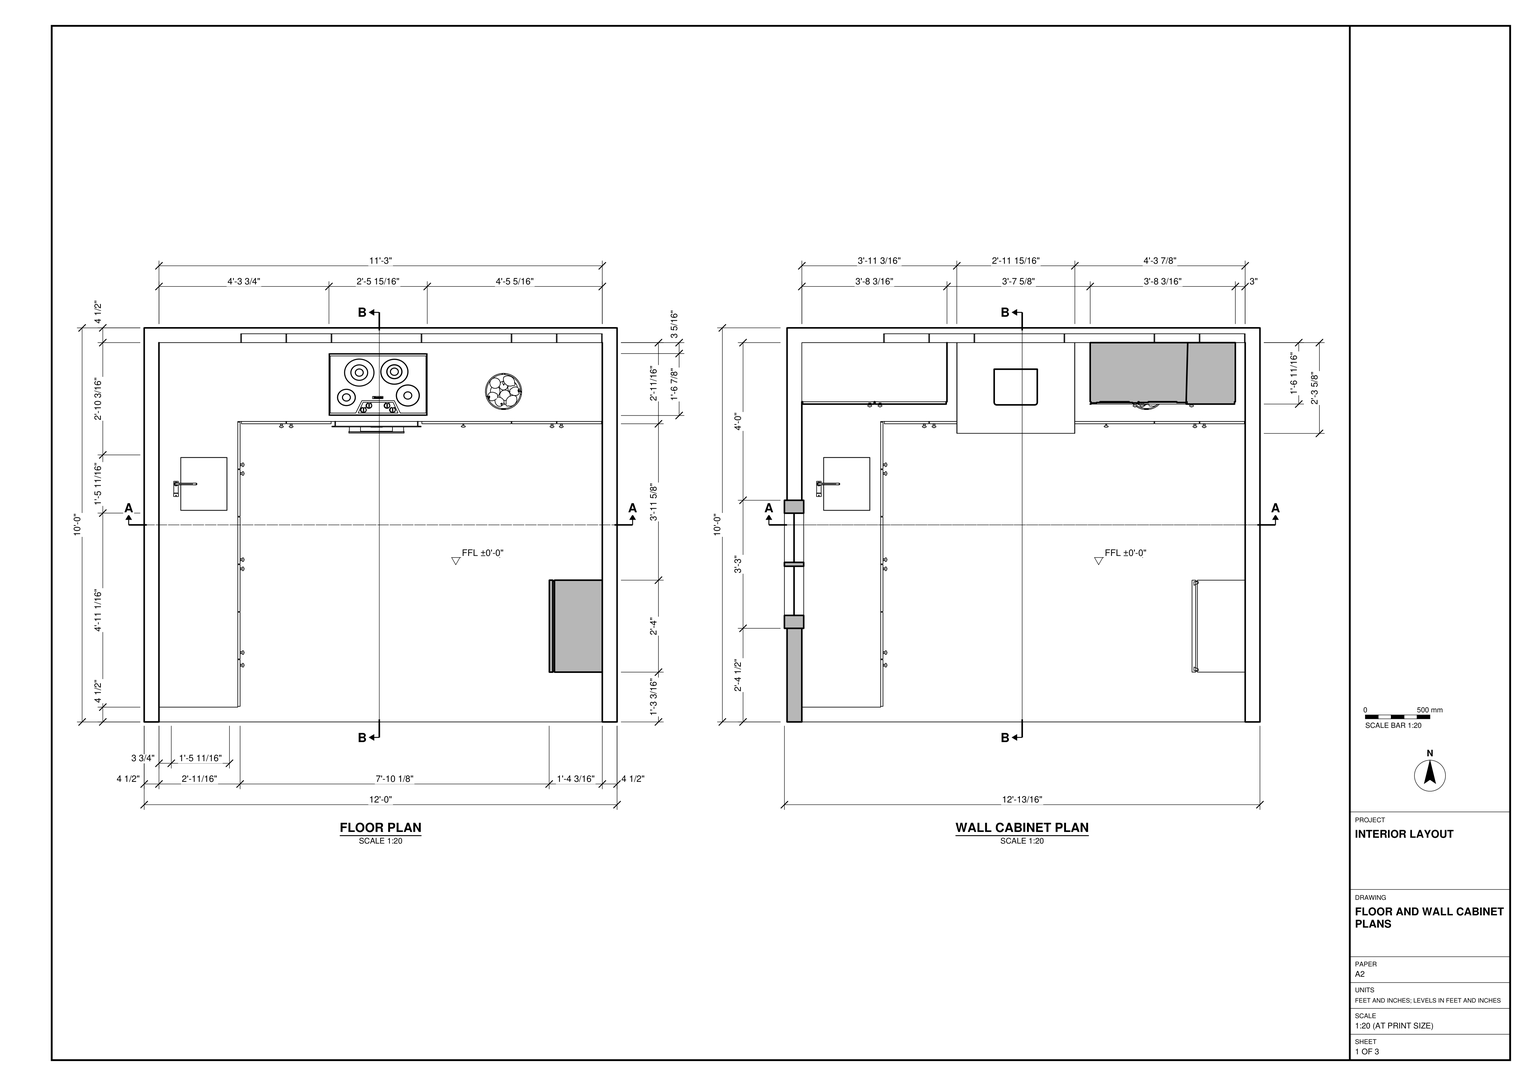
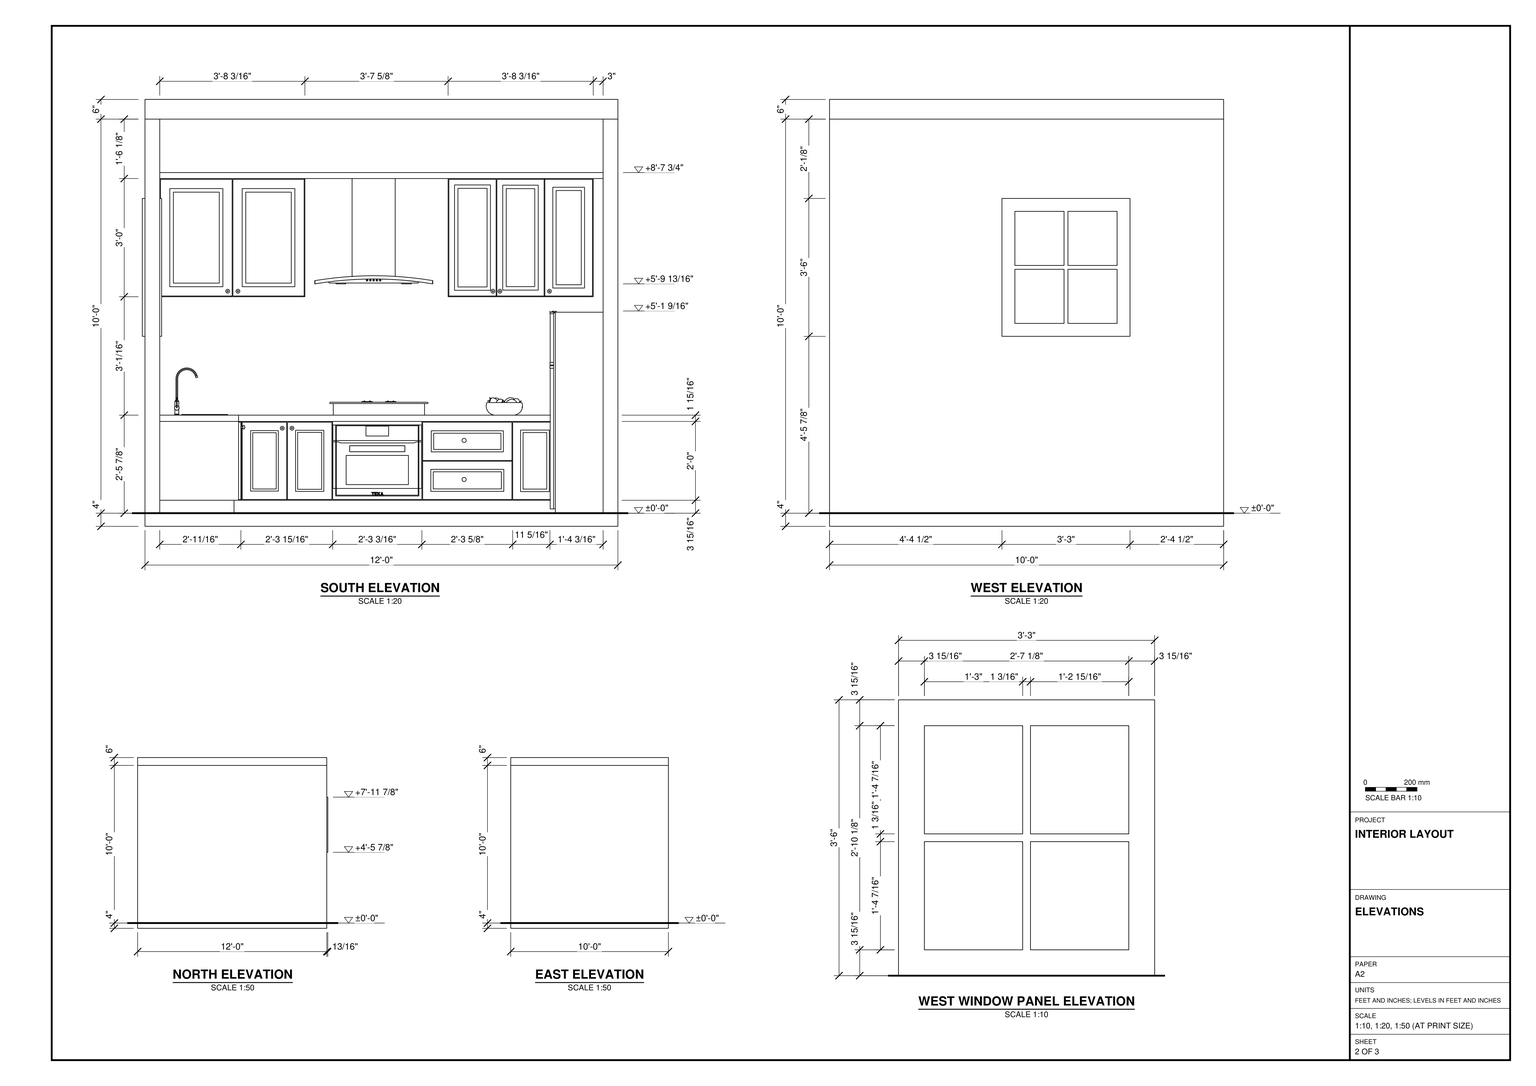
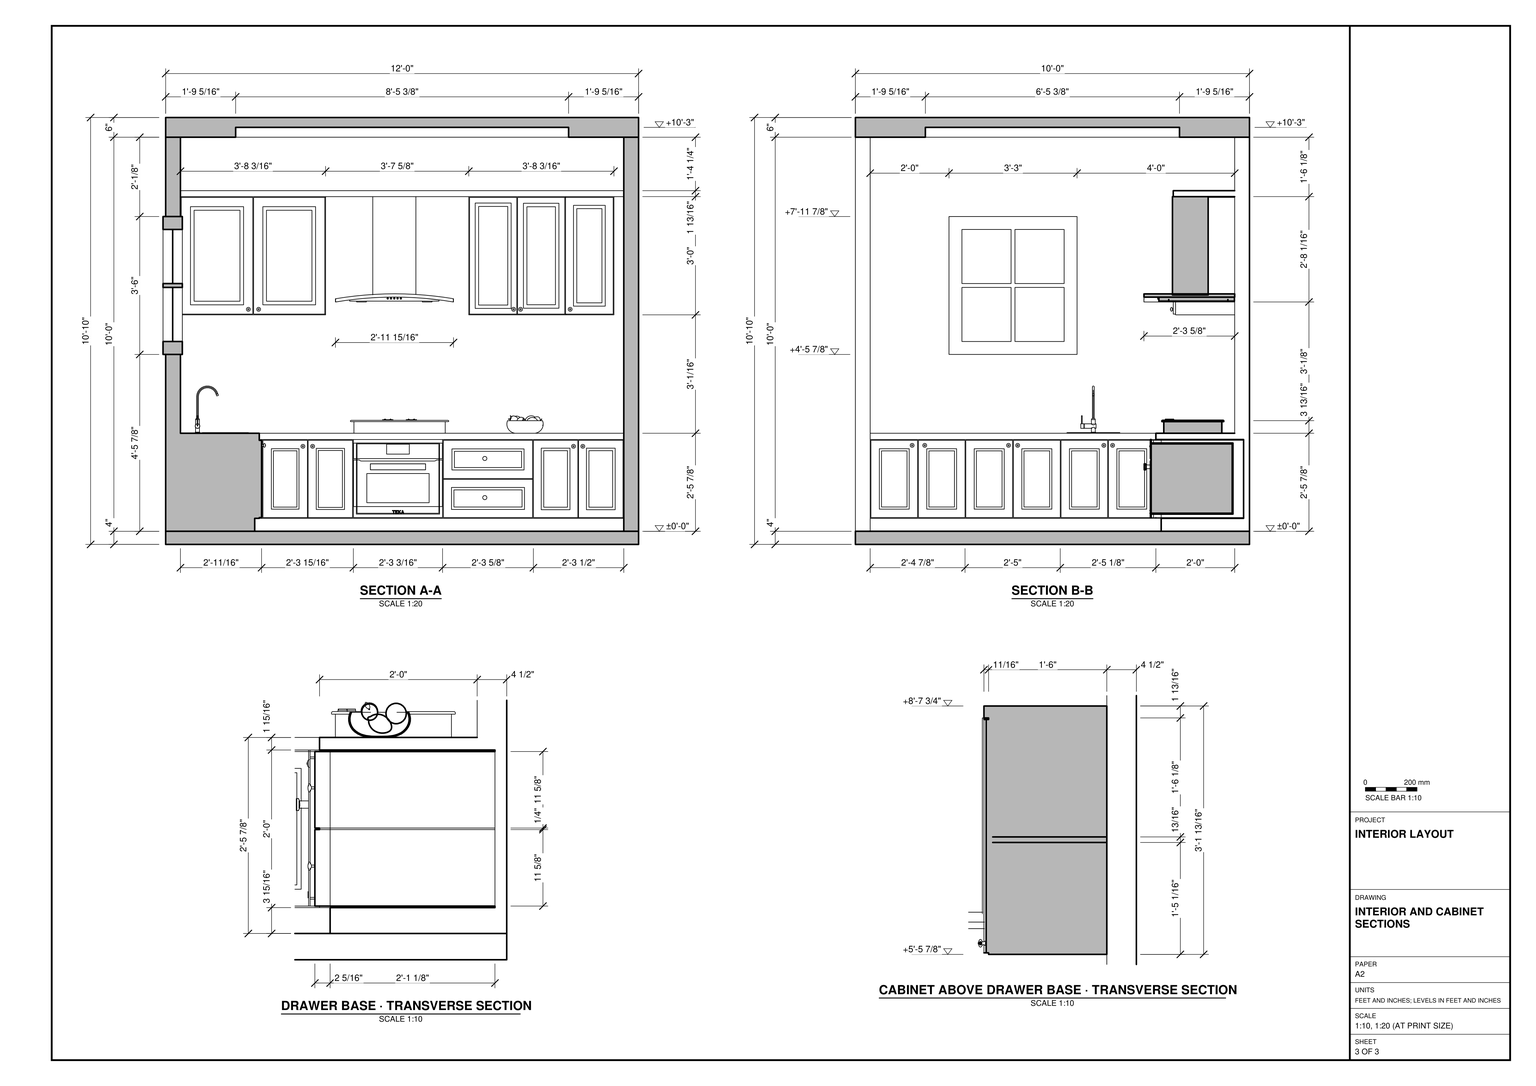
Build the kitchen in SketchUp from task_files/diagram_01.pdf. Work in feet and inches. Set the finished floor at ±0'-0" and make the overall model 12'-13/16" wide along X, 10'-0" deep along Y and 10'-10" high along Z.

Model the floor slab, the 4 1/2" back and side walls, and the roof slab with its recessed underside. Leave the front open as drawn. Use the west elevation and window detail to place the four-pane window in the side wall.

Run the base cabinets and countertop along the back wall and around the corner onto the west wall. Fit the sink and faucet into the west return. On the back run, place the cooktop over the oven, with the drawer base to its right. Mount the upper cabinets on either side of the extractor hood. Follow the elevations for the door and drawer divisions, and the cabinet sections for the countertop edge, recessed plinth and shelf above the drawer base. Place the tall appliance against the opposite side wall and the fruit bowl on the back counter. Decor and loose items, including appliances, may be any suitable library components.

Keep the walls, slabs and each joinery piece in separate groups or components, and use components for repeated parts. Save one SketchUp model as output_files/open_front_kitchen_with_l_shaped_cabinetry.skp.

# SketchUp Ruby script. Lengths in inches.
U = 1.inch
M = Sketchup.active_model
def pt(a) = Geom::Point3d.new(a.map { |v| v * U })
def face(e, loops, mat)
  f = e.add_face(loops[0].map { |a| pt(a) })
  loops[1..].each { |l| e.add_face(l.map { |a| pt(a) }).erase! }
  f.material = f.back_material = mat if mat
  f
end
# faces: each face lists its corners as indices into pts; further lists are holes
def faces(e, pts, list, mat = nil) = list.each { |f| face(e, (f[0].is_a?(Array) ? f : [f]).map { |l| l.map { |i| pts[i] } }, mat) }
# xy, xz, yz: faces in a plane at the given z, y or x. An outline is a flat list of corners, or four numbers for a rectangle; further outlines are holes
def ring(l) = l.size == 4 ? [[l[0], l[1]], [l[2], l[1]], [l[2], l[3]], [l[0], l[3]]] : l.each_slice(2).to_a
def flat(e, list, mat, &to3) = list.each { |f| face(e, (f[0].is_a?(Array) ? f : [f]).map { |l| ring(l).map { |u, v| to3.(u, v) } }, mat) }
def xy(e, z, list, mat = nil) = flat(e, list, mat) { |x, y| [x, y, z] }
def xz(e, y, list, mat = nil) = flat(e, list, mat) { |x, z| [x, y, z] }
def yz(e, x, list, mat = nil) = flat(e, list, mat) { |y, z| [x, y, z] }
def lines(e, pts, list) = list.each { |a, b| e.add_line(pt(pts[a]), pt(pts[b])) }
# prism: a flat outline (further loops are holes) pulled along v
def prism(e, loops, v, mat = nil)
  f = face(e, loops, mat); d = Geom::Vector3d.new(v.map { |x| x * U })
  f.pushpull(f.normal.samedirection?(d) ? d.length : -d.length)
end
def box(e, o, s, mat = nil) = prism(e, [[o, [o[0] + s[0], o[1], o[2]], [o[0] + s[0], o[1] + s[1], o[2]], [o[0], o[1] + s[1], o[2]]]], [0, 0, s[2]], mat)
def at(x, y, z, deg = 0) = Geom::Transformation.translation(pt([x, y, z])) * Geom::Transformation.rotation(ORIGIN, Z_AXIS, deg.degrees)
def axes(o, x, y, z) = Geom::Transformation.new([*x, 0, *y, 0, *z, 0, *pt(o).to_a, 1])
def part(name) = M.definitions.add(name)
# library, detail: a bought-in or finely detailed component or shape, given as its bounding box
def library(name, o, s) = part(name).tap { |d| box(d.entities, o, s) }
def detail(e, o, s) = box(e.add_group.entities, o, s)
def put(e, d, t, mat = nil) = e.add_instance(d, t).tap { |i| i.material = mat if mat }
def group(e, t, mat = nil) = e.add_group.tap { |g| g.transformation = t; g.material = mat if mat }.entities
root = M.entities
M.materials.add("2153 AP 7328 GREEK VASE").color = [106, 175, 217]
M.materials.add("GLASSS MICROWAVE").color = [91, 93, 94]
M.materials["GLASSS MICROWAVE"].alpha = 0.18
M.materials.add("Glass_Sky Reflection_01").color = [126, 138, 183]
M.materials["Glass_Sky Reflection_01"].alpha = 0.25
M.materials.add("H 6800 BM").color = [58, 58, 58]
M.materials.add("M05_Graphite_Haze").color = [114, 114, 114]
M.materials.add("Stainless_Steel2").color = [164, 165, 173]
M.materials.add("W142X794B75_NILAYA IMAGINE 31718 ROLL B75").color = [176, 175, 170]
M.materials.add("W143X893B75_NILAYA NEW MODERN 31803 ROLL B75").color = [67, 87, 86]
M.materials.add("W149Z635F75_NILAYA ARCHITECTURE FD25331 ROLL F75").color = [93, 116, 118]
M.materials.add("W149Z654F75_NILAYA ARCHITECTURE FD25350 ROLL F75").color = [133, 143, 147]
M.materials.add("[0015_Salmon]").color = [26, 26, 26]
c1 = library("3-PRODUITS CUISINE CLC2",[-1.54,-1.54,0],[3.08,3.08,10.36])
c2 = library("12-POIGNEE CLC2",[-0.65,-0.63,0],[1.26,1.26,1.0625])
c3 = library("11-POIGNEE CLC2",[-0.59,-0.59,0],[1.18,1.18,1.22])
c4 = library("14-PRODUITS CUISINE CLC2",[-1.97,-1.97,0],[3.94,3.94,3.9375])
c5 = library("4-PRODUITS CUISINE CLC2",[-1.73,-1.73,0],[3.46,3.46,11.45])
c6 = library("6-PRODUITS CUISINE CLC2",[-1.1,-1.1,0],[2.2,2.2,8.09])
c7 = library("TEKA\#1",[0.03,0,0],[3.05,0.72,0.08])
c8 = library("18-PRODUITS CUISINE CLC2",[-2.03,-2.03,0],[4.06,4.06,6.48])
c9 = library("7-PRODUITS CUISINE CLC2",[-1.88,-1.88,0],[3.76,3.76,5.32])
c10 = library("1-PNGFRUITS CLC2",[-5.8,-5.64,-0.15],[11.3,11.71,6.42])
c11 = library("Electric cooktop",[0,0,0],[29.93,18.87,4.33])
c12 = library("24-PRODUITS CUISINE CLC2",[-4.72,-4.72,0],[9.44,9.44,4.33])
c13 = library("13-PRODUITS CUISINE CLC2",[-1.97,-1.97,0],[3.94,3.94,3.9375])
c14 = library("1-EVIER M60 CLC2",[-8.86,-8.86,-7.68],[17.72,17.72,22.07])
c15 = library("chimney",[0,0,0],[35.95,27.65,32.08])
c16 = library("ENERGISK+B18+S (1)",[50,0,0],[28,31.125,68.4])
c17 = library("16-PRODUITS CUISINE CLC2",[-2.49,-2.49,0],[4.98,4.98,4.3])
c18 = part("Group124\#2")
xy(c18.entities,0,[[-15.5625,-17.0625,-0.59,-0.59],[0.59,-17.0625,15.5625,-0.59],[-15.5625,0.59,-0.59,17.0625],[0.59,0.59,15.5625,17.0625]])
xy(root,-4,[[0.81,0,144.81,120]])
xy(root,0,[[0.81,0,5.31,0,5.31,4.5,27.92,4.5,27.92,93.11,140.31,93.11,140.31,0,144.81,0,144.81,120,0.81,120],[5.31,0,140.31,0,140.31,93.11,27.92,93.11,27.92,4.5,5.31,4.5]],"W142X794B75_NILAYA IMAGINE 31718 ROLL B75")
xy(root,3.9375,[[27.92,4.5,29.31,91.5],[27.92,91.5,30.2,93.11],[30.2,93.11,140.31,118.21]],"W142X794B75_NILAYA IMAGINE 31718 ROLL B75")
xy(root,4.17,[[29.31,4.74,30.01,18.94],[29.31,19.18,30.01,33.38],[29.31,33.62,30.01,47.88],[29.31,48.12,30.01,62.38],[29.31,62.62,30.01,76.82],
  [29.31,77.06,30.01,91.26],[30.43,90.79,43.96,118.21],[44.2,90.79,57.72,118.21],[85.37,90.79,98.84,118.21],[98.84,90.79,99.07,118.21],
  [99.07,90.79,112.54,118.21],[112.78,90.79,126.31,118.21],[126.54,90.79,140.07,118.21],[43.96,91.5,44.2,93.11],[126.31,91.5,126.54,93.11],
  [43.96,93.11,44.2,118.21],[126.31,93.11,126.54,118.21]],"W142X794B75_NILAYA IMAGINE 31718 ROLL B75")
xy(root,15.82,[[85.37,90.79,112.54,91.5]],"W142X794B75_NILAYA IMAGINE 31718 ROLL B75")
xy(root,16.06,[[85.37,90.79,112.54,91.5]],"W142X794B75_NILAYA IMAGINE 31718 ROLL B75")
xy(root,27.7,[[30.43,90.79,43.96,118.21],[44.2,90.79,57.72,118.21],[85.37,90.79,112.54,118.21],[112.78,90.79,126.31,118.21],[126.54,90.79,140.07,118.21]],"W142X794B75_NILAYA IMAGINE 31718 ROLL B75")
xy(root,27.7,[[29.31,4.74,30.01,18.94],[29.31,19.18,30.01,33.38],[29.31,33.62,30.01,47.88],[29.31,48.12,30.01,62.38],[29.31,62.62,30.01,76.82],
  [29.31,77.06,30.01,91.26]],"W143X893B75_NILAYA NEW MODERN 31803 ROLL B75")
xy(root,27.9375,[[30.2,91.5,140.31,118.21]],"W142X794B75_NILAYA IMAGINE 31718 ROLL B75")
xy(root,29.85,[[[5.31,4.5,29.31,4.5,29.31,91.5,140.31,91.5,140.31,115.5,5.31,115.5],[11.97,64.44,25.99,80.5]]],"W142X794B75_NILAYA IMAGINE 31718 ROLL B75")
xy(root,53.85,[[0,28.5,0.81,67.5],[0.81,28.5,2.9375,67.5],[2.9375,28.5,5.07,67.5],[5.07,28.5,5.31,67.5],[5.31,28.5,5.875,67.5]],"W142X794B75_NILAYA IMAGINE 31718 ROLL B75")
xy(root,57.79,[[0,32.4375,5.875,47.41],[0,48.59,5.875,63.5625]],"M05_Graphite_Haze")
xy(root,65.91,[[93.11,97.5,137.31,115.5]],"W143X893B75_NILAYA NEW MODERN 31803 ROLL B75")
xy(root,65.91,[[5.31,97.5,49.5,115.5]],"W149Z635F75_NILAYA ARCHITECTURE FD25331 ROLL F75")
xy(root,66.14,[[93.34,96.79,107.72,97.125],[107.96,96.79,122.34,97.27],[93.34,97.125,107.72,97.5],[107.96,97.27,122.34,97.5]],"W142X794B75_NILAYA IMAGINE 31718 ROLL B75")
xy(root,66.14,[[122.57,96.79,137.07,97.5]],"W143X893B75_NILAYA NEW MODERN 31803 ROLL B75")
xy(root,66.14,[[5.54,96.79,27.34,97.5],[27.58,96.79,49.27,97.5]],"W149Z635F75_NILAYA ARCHITECTURE FD25331 ROLL F75")
xy(root,67.86,[[95.0625,97.125,106.01,97.27]],"W142X794B75_NILAYA IMAGINE 31718 ROLL B75")
xy(root,68.89,[[96.09,97.27,104.97,97.5]],"W142X794B75_NILAYA IMAGINE 31718 ROLL B75")
xy(root,68.99,[[110.8,97.27,119.49,97.5]],"W142X794B75_NILAYA IMAGINE 31718 ROLL B75")
xy(root,74.25,[[0,32.4375,5.875,47.41],[0,48.59,5.875,63.5625]],"W142X794B75_NILAYA IMAGINE 31718 ROLL B75")
xy(root,75.44,[[0,32.4375,5.875,47.41],[0,48.59,5.875,63.5625]],"M05_Graphite_Haze")
xy(root,82.94,[[93.11,97.5,93.34,97.5,93.34,98.125,107.72,98.125,107.72,97.5,107.96,97.5,107.96,98.02,122.34,98.02,122.34,97.5,122.81,97.5,122.81,115.5,93.11,115.5]],"W142X794B75_NILAYA IMAGINE 31718 ROLL B75")
xy(root,83.79,[[93.11,97.5,93.11,115.5,122.81,115.5,122.81,97.5,122.34,97.5,122.34,98.02,107.96,98.02,107.96,97.5,107.72,97.5,107.72,98.125,93.34,98.125,93.34,97.5]],"W142X794B75_NILAYA IMAGINE 31718 ROLL B75")
xy(root,91.91,[[0,32.4375,5.875,47.41],[0,48.59,5.875,63.5625]],"W142X794B75_NILAYA IMAGINE 31718 ROLL B75")
xy(root,95.85,[[0,28.5,0.81,67.5],[0.81,28.5,2.9375,67.5],[2.9375,28.5,5.07,67.5],[5.07,28.5,5.31,67.5],[5.31,28.5,5.875,67.5]],"W142X794B75_NILAYA IMAGINE 31718 ROLL B75")
xy(root,98.82,[[110.8,97.27,119.49,97.5]],"W142X794B75_NILAYA IMAGINE 31718 ROLL B75")
xy(root,98.92,[[96.09,97.27,104.97,97.5]],"W142X794B75_NILAYA IMAGINE 31718 ROLL B75")
xy(root,99.95,[[95.0625,97.125,106.01,97.27]],"W142X794B75_NILAYA IMAGINE 31718 ROLL B75")
xy(root,101.67,[[93.34,96.79,107.72,97.125],[107.96,96.79,122.34,97.27],[93.34,97.125,107.72,97.5],[107.96,97.27,122.34,97.5]],"W142X794B75_NILAYA IMAGINE 31718 ROLL B75")
xy(root,101.67,[[122.57,96.79,137.07,97.5]],"W143X893B75_NILAYA NEW MODERN 31803 ROLL B75")
xy(root,101.67,[[5.54,96.79,27.34,97.5],[27.58,96.79,49.27,97.5]],"W149Z635F75_NILAYA ARCHITECTURE FD25331 ROLL F75")
xy(root,101.91,[[5.31,96.79,49.5,97.5],[49.5,96.79,93.11,115.5],[93.11,96.79,137.31,97.5],[137.31,96.79,140.31,115.5]],"W142X794B75_NILAYA IMAGINE 31718 ROLL B75")
xy(root,103.72,[[5.31,96.79,140.31,115.5]],"2153 AP 7328 GREEK VASE")
xy(root,120,[[[5.31,0,140.31,115.5],[22.12,21.31,123.5,98.69]]])
xy(root,120,[[0.81,0,0.81,120,144.81,120,144.81,0,140.31,0,140.31,115.5,5.31,115.5,5.31,0]],"W142X794B75_NILAYA IMAGINE 31718 ROLL B75")
xy(root,123,[[22.12,21.31,123.5,98.69]])
xy(root,126,[[0.81,0,144.81,120]])
xz(root,0,[[0.81,-4,144.81,0],[0.81,120,144.81,126]])
xz(root,0,[[0.81,0,5.31,120],[140.31,0,144.81,120]],"W142X794B75_NILAYA IMAGINE 31718 ROLL B75")
xz(root,4.5,[[5.31,0,27.92,3.9375],[5.31,27.9375,29.31,29.85]],"W142X794B75_NILAYA IMAGINE 31718 ROLL B75")
xz(root,4.5,[[5.31,3.9375,29.31,27.9375]],"W143X893B75_NILAYA NEW MODERN 31803 ROLL B75")
xz(root,4.74,[[29.31,4.17,30.01,27.7]],"W143X893B75_NILAYA NEW MODERN 31803 ROLL B75")
xz(root,18.94,[[29.31,4.17,30.01,27.7]],"W142X794B75_NILAYA IMAGINE 31718 ROLL B75")
xz(root,19.18,[[29.31,4.17,30.01,27.7]],"W142X794B75_NILAYA IMAGINE 31718 ROLL B75")
xz(root,21.31,[[22.12,120,123.5,123]])
xz(root,28.5,[[0,53.85,0.81,95.85],[0.81,53.85,2.9375,95.85],[2.9375,53.85,5.07,95.85],[5.07,53.85,5.31,95.85],[5.31,53.85,5.875,95.85]],"W142X794B75_NILAYA IMAGINE 31718 ROLL B75")
xz(root,32.4375,[[0,57.79,5.875,74.25],[0,75.44,5.875,91.91]],"M05_Graphite_Haze")
xz(root,33.38,[[29.31,4.17,30.01,27.7]],"W142X794B75_NILAYA IMAGINE 31718 ROLL B75")
xz(root,33.62,[[29.31,4.17,30.01,27.7]],"W142X794B75_NILAYA IMAGINE 31718 ROLL B75")
xz(root,47.41,[[0,57.79,5.875,74.25],[0,75.44,5.875,91.91]],"M05_Graphite_Haze")
xz(root,47.88,[[29.31,4.17,30.01,27.7]],"W142X794B75_NILAYA IMAGINE 31718 ROLL B75")
xz(root,48.12,[[29.31,4.17,30.01,27.7]],"W142X794B75_NILAYA IMAGINE 31718 ROLL B75")
xz(root,48.59,[[0,57.79,5.875,74.25],[0,75.44,5.875,91.91]],"W142X794B75_NILAYA IMAGINE 31718 ROLL B75")
xz(root,62.38,[[29.31,4.17,30.01,27.7]],"W142X794B75_NILAYA IMAGINE 31718 ROLL B75")
xz(root,62.62,[[29.31,4.17,30.01,27.7]],"W142X794B75_NILAYA IMAGINE 31718 ROLL B75")
xz(root,63.5625,[[0,57.79,5.875,74.25],[0,75.44,5.875,91.91]],"M05_Graphite_Haze")
xz(root,67.5,[[0,53.85,0.81,95.85],[0.81,53.85,2.9375,95.85],[2.9375,53.85,5.07,95.85],[5.07,53.85,5.31,95.85],[5.31,53.85,5.875,95.85]],"W142X794B75_NILAYA IMAGINE 31718 ROLL B75")
xz(root,76.82,[[29.31,4.17,30.01,27.7]],"W142X794B75_NILAYA IMAGINE 31718 ROLL B75")
xz(root,77.06,[[29.31,4.17,30.01,27.7]],"W142X794B75_NILAYA IMAGINE 31718 ROLL B75")
xz(root,90.79,[[[115.17,6.5625,123.91,25.31],[115.93,7.33,123.15,24.54]],[[128.93,6.5625,137.68,25.31],[129.7,7.33,136.91,24.54]],[[46.66,6.63,55.26,25.24],[47.29,7.27,54.63,24.61]],[[87.84,6.65,110.07,13.35],[88.58,7.39,109.33,12.6]],[[32.99,6.73,41.4,25.14],[33.62,7.36,40.77,24.51]],
  [[87.98,18.67,109.93,25.09],[88.72,19.41,109.1875,24.35]]])
xz(root,90.79,[[[30.43,4.17,43.96,27.7],[32.99,6.73,41.4,25.14]],[[44.2,4.17,57.72,27.7],[46.66,6.63,55.26,25.24]],[[85.37,4.17,112.54,15.82],[87.84,6.65,110.07,13.35]],[[112.78,4.17,126.31,27.7],[115.17,6.5625,123.91,25.31]],[[126.54,4.17,140.07,27.7],[128.93,6.5625,137.68,25.31]],
  [47.29,7.27,54.63,24.61],[115.93,7.33,123.15,24.54],[129.7,7.33,136.91,24.54],[33.62,7.36,40.77,24.51],[88.58,7.39,109.33,12.6],
  [[85.37,16.06,112.54,27.7],[87.98,18.67,109.93,25.09]],[88.72,19.41,109.1875,24.35]],"W143X893B75_NILAYA NEW MODERN 31803 ROLL B75")
xz(root,91.26,[[29.31,4.17,30.01,27.7]],"W142X794B75_NILAYA IMAGINE 31718 ROLL B75")
xz(root,91.5,[[29.31,3.9375,30.2,27.9375],[85.37,15.82,112.54,16.06],[29.31,27.9375,140.31,29.85]],"W142X794B75_NILAYA IMAGINE 31718 ROLL B75")
xz(root,93.11,[[27.92,0,140.31,3.9375]],"W142X794B75_NILAYA IMAGINE 31718 ROLL B75")
xz(root,96.79,[[[124.99,68.56,134.65,99.25],[125.99,69.56,133.65,98.25]],[[8.36,68.96,24.53,98.85],[9.46,70.06,23.43,97.75]],[[30.4,68.96,46.45,98.85],[31.5,70.06,45.35,97.75]]])
xz(root,96.79,[[5.31,101.91,140.31,103.72]],"2153 AP 7328 GREEK VASE")
xz(root,96.79,[[93.11,66.14,93.34,66.14,93.34,101.67,107.72,101.67,107.72,66.14,107.96,66.14,107.96,101.67,122.57,101.67,122.57,101.91,93.11,101.91],[122.34,66.14,122.57,101.67]],"W142X794B75_NILAYA IMAGINE 31718 ROLL B75")
xz(root,96.79,[[[122.57,66.14,137.07,101.67],[124.99,68.56,134.65,99.25]],[125.99,69.56,133.65,98.25]],"W143X893B75_NILAYA NEW MODERN 31803 ROLL B75")
xz(root,96.79,[[[5.54,66.14,27.34,101.67],[8.36,68.96,24.53,98.85]],[[27.58,66.14,49.27,101.67],[30.4,68.96,46.45,98.85]],[9.46,70.06,23.43,97.75],[31.5,70.06,45.35,97.75]],"W149Z635F75_NILAYA ARCHITECTURE FD25331 ROLL F75")
xz(root,97.125,[[[93.34,66.14,107.72,101.67],[95.0625,67.86,106.01,99.95]]],"W143X893B75_NILAYA NEW MODERN 31803 ROLL B75")
xz(root,97.27,[[[95.0625,67.86,106.01,99.95],[96.09,68.89,104.97,98.92]],[[109.74,67.93,120.55,99.88],[110.8,68.99,119.49,98.82]]])
xz(root,97.27,[[[107.96,66.14,122.34,101.67],[109.74,67.93,120.55,99.88]]],"W143X893B75_NILAYA NEW MODERN 31803 ROLL B75")
xz(root,97.5,[[96.09,68.89,104.97,98.92],[110.8,68.99,119.49,98.82]],"Glass_Sky Reflection_01")
xz(root,97.5,[[93.11,66.14,93.34,82.94],[93.11,82.94,93.34,83.79],[122.34,82.94,122.57,83.79],[122.57,82.94,122.81,83.79],[93.11,83.79,93.34,101.67]],"W142X794B75_NILAYA IMAGINE 31718 ROLL B75")
xz(root,97.5,[[93.11,65.91,137.31,65.91,137.31,101.91,122.34,101.91,122.34,83.79,122.57,83.79,122.57,101.67,137.07,101.67,137.07,66.14,122.57,66.14,122.57,82.94,122.34,82.94,122.34,66.14,107.96,66.14,107.96,82.94,107.72,82.94,107.72,66.14,93.11,66.14],[107.72,82.94,107.96,83.79],[107.72,83.79,107.96,83.79,107.96,101.67,122.34,101.67,122.34,101.91,93.11,101.91,93.11,101.67,107.72,101.67]],"W143X893B75_NILAYA NEW MODERN 31803 ROLL B75")
xz(root,97.5,[[[5.31,65.91,49.5,65.91,49.5,66.14,27.58,66.14,27.58,101.67,49.5,101.67,49.5,101.91,5.31,101.91],[5.54,66.14,27.34,101.67]],[49.27,66.14,49.5,101.67]],"W149Z635F75_NILAYA ARCHITECTURE FD25331 ROLL F75")
xz(root,98.02,[[107.96,82.94,122.34,83.79]],"W142X794B75_NILAYA IMAGINE 31718 ROLL B75")
xz(root,98.69,[[22.12,120,123.5,123]])
xz(root,115.5,[[93.11,65.91,122.81,82.94],[122.81,65.91,137.31,103.72],[93.11,82.94,122.81,83.79],[93.11,83.79,122.81,103.72]],"W142X794B75_NILAYA IMAGINE 31718 ROLL B75")
xz(root,118.21,[[[30.2,3.9375,140.31,27.9375],[85.37,4.17,112.54,27.7],[112.78,4.17,112.78,27.7,126.31,27.7,126.31,4.17,126.54,4.17,126.54,27.7,140.07,27.7,140.07,4.17],[30.43,4.17,30.43,27.7,43.96,27.7,43.96,4.17,44.2,4.17,44.2,27.7,57.72,27.7,57.72,4.17]]],"W142X794B75_NILAYA IMAGINE 31718 ROLL B75")
xz(root,120,[[0.81,-4,144.81,0],[0.81,120,144.81,126]])
xz(root,120,[[0.81,0,144.81,120]],"W149Z654F75_NILAYA ARCHITECTURE FD25350 ROLL F75")
yz(root,0,[[[28.5,53.85,67.5,95.85],[32.4375,75.44,47.41,91.91],[48.59,75.44,63.5625,91.91],[48.59,57.79,63.5625,74.25],[32.4375,57.79,47.41,74.25]]],"W142X794B75_NILAYA IMAGINE 31718 ROLL B75")
yz(root,0.81,[[0,-4,120,0],[0,120,120,126]])
yz(root,0.81,[[[0,0,120,120],[28.5,53.85,67.5,95.85]]],"W142X794B75_NILAYA IMAGINE 31718 ROLL B75")
yz(root,5.31,[[[4.5,29.85,115.5,29.85,115.5,65.91,97.5,65.91,97.5,101.91,96.79,101.91,96.79,103.72,115.5,103.72,115.5,120,4.5,120],[28.5,53.85,67.5,95.85]]],"2153 AP 7328 GREEK VASE")
yz(root,5.31,[[0,0,4.5,120]],"W142X794B75_NILAYA IMAGINE 31718 ROLL B75")
yz(root,5.54,[[96.79,66.14,97.5,101.67]],"W142X794B75_NILAYA IMAGINE 31718 ROLL B75")
yz(root,5.875,[[[28.5,53.85,67.5,95.85],[48.59,57.79,63.5625,74.25],[32.4375,57.79,47.41,74.25],[32.4375,75.44,47.41,91.91],[48.59,75.44,63.5625,91.91]]],"M05_Graphite_Haze")
yz(root,22.12,[[21.31,120,98.69,123]])
yz(root,27.34,[[96.79,66.14,97.5,101.67]],"W149Z635F75_NILAYA ARCHITECTURE FD25331 ROLL F75")
yz(root,27.58,[[96.79,66.14,97.5,101.67]],"W149Z635F75_NILAYA ARCHITECTURE FD25331 ROLL F75")
yz(root,27.92,[[4.5,0,93.11,3.9375]],"W142X794B75_NILAYA IMAGINE 31718 ROLL B75")
yz(root,29.31,[[[4.5,3.9375,91.5,27.9375],[33.62,4.17,47.88,27.7],[48.12,4.17,62.38,27.7],[4.74,4.17,18.94,27.7],[62.62,4.17,76.82,27.7],[19.18,4.17,33.38,27.7],[77.06,4.17,91.26,27.7]],[4.5,27.9375,91.5,29.85]],"W142X794B75_NILAYA IMAGINE 31718 ROLL B75")
yz(root,30.01,[[[7.3,6.74,16.38,25.14],[7.96,7.39,15.72,24.48]],[[21.74,6.74,30.82,25.14],[22.4,7.39,30.16,24.48]],[[36.18,6.74,45.32,25.14],[36.84,7.39,44.66,24.48]],[[50.68,6.74,59.82,25.14],[51.34,7.39,59.16,24.48]],[[65.18,6.74,74.26,25.14],[65.84,7.39,73.6,24.48]],
  [[79.62,6.74,88.7,25.14],[80.28,7.39,88.04,24.48]]])
yz(root,30.01,[[[4.74,4.17,18.94,27.7],[7.3,6.74,16.38,25.14]],[[19.18,4.17,33.38,27.7],[21.74,6.74,30.82,25.14]],[[33.62,4.17,47.88,27.7],[36.18,6.74,45.32,25.14]],[[48.12,4.17,62.38,27.7],[50.68,6.74,59.82,25.14]],[[62.62,4.17,76.82,27.7],[65.18,6.74,74.26,25.14]],
  [[77.06,4.17,91.26,27.7],[79.62,6.74,88.7,25.14]],[7.96,7.39,15.72,24.48],[22.4,7.39,30.16,24.48],[36.84,7.39,44.66,24.48],[51.34,7.39,59.16,24.48],
  [65.84,7.39,73.6,24.48],[80.28,7.39,88.04,24.48]],"W143X893B75_NILAYA NEW MODERN 31803 ROLL B75")
yz(root,30.2,[[91.5,3.9375,118.21,27.9375]],"W142X794B75_NILAYA IMAGINE 31718 ROLL B75")
yz(root,30.43,[[90.79,4.17,118.21,27.7]],"W142X794B75_NILAYA IMAGINE 31718 ROLL B75")
yz(root,43.96,[[90.79,4.17,118.21,27.7]],"W142X794B75_NILAYA IMAGINE 31718 ROLL B75")
yz(root,44.2,[[90.79,4.17,118.21,27.7]],"W142X794B75_NILAYA IMAGINE 31718 ROLL B75")
yz(root,49.27,[[96.79,66.14,97.5,101.67]],"W149Z635F75_NILAYA ARCHITECTURE FD25331 ROLL F75")
yz(root,49.5,[[97.5,65.91,115.5,101.67]],"W149Z635F75_NILAYA ARCHITECTURE FD25331 ROLL F75")
yz(root,57.72,[[90.79,4.17,118.21,27.7]],"W142X794B75_NILAYA IMAGINE 31718 ROLL B75")
yz(root,57.96,[[93.11,4.17,118.21,27.7]],"W142X794B75_NILAYA IMAGINE 31718 ROLL B75")
yz(root,85.13,[[93.11,4.17,118.21,27.7]],"W142X794B75_NILAYA IMAGINE 31718 ROLL B75")
yz(root,85.37,[[90.79,4.17,118.21,15.82],[91.5,15.82,118.21,16.06],[90.79,16.06,118.21,27.7]],"W142X794B75_NILAYA IMAGINE 31718 ROLL B75")
yz(root,93.11,[[97.5,101.67,115.5,101.91]],"W142X794B75_NILAYA IMAGINE 31718 ROLL B75")
yz(root,93.11,[[97.5,65.91,115.5,82.94],[97.5,82.94,115.5,83.79],[97.5,83.79,115.5,101.67]],"W143X893B75_NILAYA NEW MODERN 31803 ROLL B75")
yz(root,93.34,[[96.79,66.14,97.125,101.67],[97.125,66.14,97.5,82.94],[97.125,82.94,97.5,83.79],[97.5,82.94,98.125,83.79],[97.125,83.79,97.5,101.67]],"W142X794B75_NILAYA IMAGINE 31718 ROLL B75")
yz(root,95.0625,[[97.125,67.86,97.27,82.94],[97.125,82.94,97.27,83.79],[97.125,83.79,97.27,99.95]],"W142X794B75_NILAYA IMAGINE 31718 ROLL B75")
yz(root,96.09,[[97.27,68.89,97.5,82.94],[97.27,82.94,97.5,83.79],[97.27,83.79,97.5,98.92]],"W142X794B75_NILAYA IMAGINE 31718 ROLL B75")
yz(root,104.97,[[97.27,68.89,97.5,82.94],[97.27,82.94,97.5,83.79],[97.27,83.79,97.5,98.92]],"W142X794B75_NILAYA IMAGINE 31718 ROLL B75")
yz(root,106.01,[[97.125,67.86,97.27,82.94],[97.125,82.94,97.27,83.79],[97.125,83.79,97.27,99.95]],"W142X794B75_NILAYA IMAGINE 31718 ROLL B75")
yz(root,107.72,[[96.79,66.14,97.125,101.67],[97.125,66.14,97.5,82.94],[97.125,82.94,97.5,83.79],[97.5,82.94,98.125,83.79],[97.125,83.79,97.5,101.67]],"W142X794B75_NILAYA IMAGINE 31718 ROLL B75")
yz(root,107.96,[[96.79,66.14,97.27,101.67],[97.27,66.14,97.5,82.94],[97.27,82.94,97.5,83.79],[97.5,82.94,98.02,83.79],[97.27,83.79,97.5,101.67]],"W142X794B75_NILAYA IMAGINE 31718 ROLL B75")
yz(root,110.8,[[97.27,68.99,97.5,82.94],[97.27,82.94,97.5,83.79],[97.27,83.79,97.5,98.82]],"W142X794B75_NILAYA IMAGINE 31718 ROLL B75")
yz(root,112.54,[[90.79,4.17,118.21,15.82],[91.5,15.82,118.21,16.06],[90.79,16.06,118.21,27.7]],"W142X794B75_NILAYA IMAGINE 31718 ROLL B75")
yz(root,112.78,[[90.79,4.17,118.21,27.7]],"W142X794B75_NILAYA IMAGINE 31718 ROLL B75")
yz(root,119.49,[[97.27,68.99,97.5,82.94],[97.27,82.94,97.5,83.79],[97.27,83.79,97.5,98.82]],"W142X794B75_NILAYA IMAGINE 31718 ROLL B75")
yz(root,122.34,[[96.79,66.14,97.27,101.67],[97.27,66.14,97.5,82.94],[97.27,82.94,97.5,83.79],[97.5,82.94,98.02,83.79],[97.27,83.79,97.5,101.67]],"W142X794B75_NILAYA IMAGINE 31718 ROLL B75")
yz(root,122.57,[[96.79,66.14,97.5,101.67]],"W143X893B75_NILAYA NEW MODERN 31803 ROLL B75")
yz(root,122.81,[[97.5,82.94,115.5,83.79]],"W142X794B75_NILAYA IMAGINE 31718 ROLL B75")
yz(root,123.5,[[21.31,120,98.69,123]])
yz(root,126.31,[[90.79,4.17,118.21,27.7]],"W142X794B75_NILAYA IMAGINE 31718 ROLL B75")
yz(root,126.54,[[90.79,4.17,118.21,27.7]],"W142X794B75_NILAYA IMAGINE 31718 ROLL B75")
yz(root,137.07,[[96.79,66.14,97.5,101.67]],"W143X893B75_NILAYA NEW MODERN 31803 ROLL B75")
yz(root,137.31,[[97.5,65.91,115.5,101.91]],"W143X893B75_NILAYA NEW MODERN 31803 ROLL B75")
yz(root,140.07,[[90.79,4.17,118.21,27.7]],"W142X794B75_NILAYA IMAGINE 31718 ROLL B75")
yz(root,140.31,[[4.5,0,4.5,120,115.5,120,115.5,103.72,96.79,103.72,96.79,101.91,115.5,101.91,115.5,29.85,91.5,29.85,91.5,27.9375,118.21,27.9375,118.21,3.9375,93.11,3.9375,93.11,0]],"2153 AP 7328 GREEK VASE")
yz(root,140.31,[[0,0,4.5,120]],"W142X794B75_NILAYA IMAGINE 31718 ROLL B75")
yz(root,144.81,[[0,-4,120,0],[0,120,120,126]])
yz(root,144.81,[[0,0,120,120]],"W142X794B75_NILAYA IMAGINE 31718 ROLL B75")
p = [[122.34,97.5,66.14],[122.81,115.5,65.91],[122.81,115.5,66.14],[122.81,115.5,82.94],[122.81,115.5,83.79],[122.81,115.5,101.67],
  [122.34,97.5,101.67],[122.34,97.5,83.79],[122.34,97.5,82.94],[10.16,71.98,32.63],[10.2,71.94,32.65],[10.08,72.04,32.57],
  [9.99,72.75,31.59],[10.01,72.78,31.55],[10.32,73.01,31.375],[10.35,73.02,31.37],[10.35,73.02,32.7],[10.32,73.01,32.7],
  [10.65,71.88,32.7],[10.5,71.86,32.72],[10.08,72.87,31.5],[10.5,73.04,32.72],[10.08,72.04,31.5],[10.01,72.12,31.55],
  [10.16,72.93,31.44],[10.2,72.96,31.42],[10.32,71.89,32.7],[10.2,71.94,31.42],[10.16,71.98,31.44],[10.5,73.04,31.35],
  [10.65,73.02,31.37],[10.16,72.93,32.63],[10.08,72.87,32.57],[9.99,72.16,31.59],[9.93,72.3,31.66],[10.5,71.86,31.35],
  [10.35,71.88,31.37],[9.93,72.61,31.66],[10.32,71.89,31.375],[10.35,71.88,32.7],[10.85,71.98,32.63],[10.8,71.94,32.65],
  [11.07,72.61,34],[11.02,72.75,34],[10.92,72.87,34],[10.8,72.96,34],[10.65,73.02,34],[9.91,72.45,32.38],
  [9.93,72.3,32.41],[10.8,72.96,32.65],[10.85,72.93,32.63],[10.2,72.96,32.65],[10.01,72.78,32.52],[10.68,73.01,32.7],
  [10.5,73.04,34],[10.35,73.02,34],[10.2,72.96,34],[9.93,72.61,32.41],[10.85,69.7,31.44],[10.99,69.7,31.55],
  [9.99,72.16,32.48],[10.01,72.12,32.52],[9.91,72.45,31.69],[10.68,71.89,32.7],[10.65,73.02,32.7],[9.99,72.75,32.48],
  [10.95,69.62,31.58],[11.06,69.62,31.72],[11.12,69.62,32.2],[11.06,69.62,32.35],[10.82,69.62,32.59],[10.67,69.62,32.65],
  [9.88,69.62,32.2],[9.86,69.62,32.03],[10.5,69.7,31.35],[10.68,69.7,31.375],[10.01,69.7,32.52],[9.9,69.7,32.38],
  [9.84,69.7,32.21],[9.8125,69.7,32.03],[10.5,69.62,32.67],[10.18,69.62,31.48],[10.33,69.62,31.42],[10.18,69.62,32.59],
  [10.05,69.62,32.49],[9.95,69.62,32.35],[10.32,69.7,32.7],[10.16,69.7,32.63],[10.5,69.62,31.4],[9.9,69.7,31.69],
  [10.01,69.7,31.55],[10.95,69.62,32.49],[10.16,69.7,31.44],[11.14,69.62,32.03],[10.82,69.62,31.48],[10.67,69.62,31.42],
  [11.1,69.7,31.69],[11.17,69.7,31.86],[9.95,69.62,31.72],[10.05,69.62,31.58],[9.84,69.7,31.86],[11.12,69.62,31.87],
  [10.33,69.62,32.65],[9.88,69.62,31.87],[10.32,69.7,31.375],[10.62,68.98,32.73],[10.62,68.95,32.73],[10.56,68.85,32.74],
  [10.53,68.83,32.74],[10.42,68.87,32.73],[10.4,68.89,32.73],[10.5,69.7,32.72],[10.38,68.95,32.73],[10.39,68.98,32.73],
  [10.5,68.83,32.74],[10.47,68.83,32.74],[10.44,68.85,32.74],[10.39,68.92,32.73],[10.5,69.07,32.74],[10.53,69.0625,32.74],
  [10.58,68.87,32.73],[10.56,69.05,32.74],[10.58,69.03,32.73],[10.6,68.89,32.73],[10.4,69.01,32.73],[10.42,69.03,32.73],
  [10.6,69.01,32.73],[10.47,69.0625,32.74],[10.44,69.05,32.74],[10.62,68.92,32.73],[11.9375,80.54,30.05],[11.9375,64.4,30.05],
  [26.03,80.54,30.05],[9.93,72.3,34],[9.99,72.16,34],[11.02,72.16,34],[11.07,72.3,34],[10.5,71.86,34],
  [10.65,71.88,34],[11.09,72.45,34],[11.1,69.7,32.38],[10.99,69.7,32.52],[10.2,71.94,34],[10.35,71.88,34],
  [10.8,71.94,34],[26.03,64.4,30.05],[10.85,69.7,32.63],[9.91,72.45,34],[11.1875,69.7,32.03],[11.17,69.7,32.21],
  [10.92,72.04,34],[10.08,72.87,34],[9.99,72.75,34],[10.68,69.7,32.7],[9.93,72.61,34],[10.08,72.04,34],
  [10.78,72.45,34.36],[10.77,72.38,34.36],[10.23,72.52,34.36],[10.26,72.59,34.36],[10.64,72.69,34.36],[10.7,72.65,34.36],
  [10.43,72.1875,34.36],[10.36,72.21,34.36],[10.43,72.72,34.36],[10.5,72.73,34.36],[10.74,72.59,34.36],[10.74,72.32,34.36],
  [10.7,72.26,34.36],[10.64,72.21,34.36],[10.77,72.52,34.36],[10.3,72.26,34.36],[10.57,72.72,34.36],[10.26,72.32,34.36],
  [10.23,72.38,34.36],[16.18,72.45,41.65],[16.19,72.52,41.65],[16.44,72.73,41.75],[16.51,72.72,41.77],[16.57,72.69,41.8],
  [16.26,72.65,41.68],[16.3125,72.69,41.7],[10.5,72.18,34.36],[16.375,72.72,41.72],[16.26,72.26,41.68],[16.22,72.32,41.66],
  [10.3,72.65,34.36],[10.36,72.69,34.36],[16.51,72.1875,41.77],[16.44,72.18,41.75],[16.625,72.65,41.82],[16.19,72.38,41.65],
  [16.7,72.45,41.85],[16.69,72.38,41.85],[16.66,72.32,41.84],[16.625,72.26,41.82],[16.66,72.59,41.84],[16.57,72.21,41.8],
  [10.22,72.45,34.36],[10.5,72.73,32.72],[10.5,72.18,32.72],[16.69,72.52,41.85],[10.57,72.1875,34.36],[16.22,72.59,41.66],
  [16.375,72.1875,41.72],[16.3125,72.21,41.7],[11.07,72.61,31.66],[11.09,72.45,31.69],[10.99,72.12,31.55],[11.02,72.16,31.59],
  [11.02,72.75,31.59],[11.07,72.3,31.66],[10.85,72.93,31.44],[10.8,72.96,31.42],[10.92,72.87,31.5],[10.99,72.78,31.55],
  [10.68,73.01,31.375],[10.85,71.98,31.44],[10.92,72.04,31.5],[10.68,71.89,31.375],[10.8,71.94,31.42],[10.65,71.88,31.37],
  [10.92,72.87,32.57],[10.99,72.78,32.52],[11.02,72.16,32.48],[10.99,72.12,32.52],[11.07,72.3,32.41],[10.92,72.04,32.57],
  [11.07,72.61,32.41],[11.09,72.45,32.38],[11.02,72.75,32.48],[57.96,93.11,4.17],[85.13,93.11,4.17]]
faces(root,p,[[0,1,2],[0,2,3,4,5,6,7,8]],"W142X794B75_NILAYA IMAGINE 31718 ROLL B75")
lines(root,p,[[9,10],[11,9],[12,13],[14,15],[16,17],[18,19],[13,20],[21,16],[22,23],[24,25],[10,26],[27,28],
  [29,30],[31,32],[33,34],[35,36],[37,12],[38,27],[39,19],[40,41],[42,43],[44,45],[45,46],[43,44],
  [47,48],[49,50],[51,31],[32,52],[15,29],[26,39],[53,49],[54,55],[55,56],[25,14],[46,54],[57,47],
  [58,59],[48,60],[61,11],[23,33],[34,62],[63,18],[41,63],[64,53],[52,65],[62,37],[17,51],[65,57],
  [20,24],[36,38],[64,21],[60,61],[28,22],[66,67],[68,69],[70,71],[72,73],[74,75],[76,77],[78,79],
  [71,80],[81,82],[83,84],[77,78],[84,85],[86,87],[82,88],[75,58],[89,90],[91,70],[90,92],[93,68],
  [94,66],[95,94],[96,97],[98,99],[79,100],[99,81],[59,96],[101,93],[80,102],[73,103],[102,83],[87,76],
  [88,95],[103,98],[92,104],[85,72],[104,74],[69,91],[100,89],[67,101],[105,106],[107,108],[109,110],[111,86],
  [112,113],[114,115],[116,109],[117,112],[118,119],[115,116],[120,107],[119,121],[121,122],[123,120],[113,124],[124,125],
  [122,126],[108,114],[127,118],[110,117],[128,127],[126,105],[125,128],[106,129],[129,123],[130,131],[132,130],[133,134],
  [135,136],[137,138],[136,139],[140,141],[142,143],[138,144],[131,145],[141,146],[147,133],[148,149],[143,137],[144,150],
  [145,132],[97,148],[149,140],[151,152],[56,151],[146,153],[152,154],[150,135],[155,142],[156,157],[134,155],[158,159],
  [154,147],[160,161],[162,163],[164,165],[161,166],[157,167],[168,169],[166,170],[163,171],[165,172],[173,174],[175,176],
  [177,178],[178,179],[180,181],[182,162],[181,183],[184,185],[186,187],[183,177],[188,189],[179,190],[185,191],[192,193],
  [194,195],[190,196],[195,197],[174,198],[199,200],[159,186],[198,158],[171,173],[196,201],[197,188],[169,202],[172,160],
  [170,156],[167,168],[187,164],[202,182],[176,203],[201,192],[193,194],[204,205],[189,204],[203,180],[205,184],[191,175],
  [153,111],[206,207],[208,209],[206,210],[209,211],[211,207],[212,213],[214,215],[213,216],[217,218],[216,30],[215,210],
  [219,220],[218,208],[35,221],[221,219],[220,217],[139,42],[212,214],[50,222],[222,223],[224,225],[226,224],[225,227],
  [228,229],[230,228],[229,226],[227,40],[223,230],[231,232]])
put(root,c1,at(98.5,106.87,83.79),"W142X794B75_NILAYA IMAGINE 31718 ROLL B75")
put(root,c2,axes([97.98,90.8,22.17],[-0.99985,0.01758,0],[0,0,1],[-0.01758,-0.99985,0]),"W142X794B75_NILAYA IMAGINE 31718 ROLL B75")
put(root,c2,axes([97.98,90.8,10.26],[-0.99985,0.01758,0],[0,0,1],[-0.01758,-0.99985,0]),"W142X794B75_NILAYA IMAGINE 31718 ROLL B75")
put(root,c3,axes([125.01,90.8,25.875],[-0.99985,0.01758,0],[0,0,1],[-0.01758,-0.99985,0]),"W142X794B75_NILAYA IMAGINE 31718 ROLL B75")
put(root,c3,axes([45.57,90.8,25.875],[-0.99985,0.01758,0],[0,0,1],[-0.01758,-0.99985,0]),"W142X794B75_NILAYA IMAGINE 31718 ROLL B75")
put(root,c3,axes([127.84,90.8,25.875],[-0.99985,0.01758,0],[0,0,1],[-0.01758,-0.99985,0]),"W143X893B75_NILAYA NEW MODERN 31803 ROLL B75")
put(root,c3,axes([42.61,90.8,25.875],[-0.99985,0.01758,0],[0,0,1],[-0.01758,-0.99985,0]),"W142X794B75_NILAYA IMAGINE 31718 ROLL B75")
put(root,c4,at(115.43,107.22,65.91),"W142X794B75_NILAYA IMAGINE 31718 ROLL B75")
put(root,c5,at(101.95,106.26,83.79),"W142X794B75_NILAYA IMAGINE 31718 ROLL B75")
put(root,c6,at(98.1,107.65,65.91),"W142X794B75_NILAYA IMAGINE 31718 ROLL B75")
put(root,c3,axes([30.01,17.27,26.17],[0,-1,0],[0,0,1],[1,0,0]),"W142X794B75_NILAYA IMAGINE 31718 ROLL B75")
put(root,c3,axes([30.01,21.11,26.17],[0,-1,0],[0,0,1],[1,0,0]),"W142X794B75_NILAYA IMAGINE 31718 ROLL B75")
put(root,c7,axes([69.8,89.84,5.42],[1.15,0,0],[0,0,1.34133],[0,-1.15,0]),"Stainless_Steel2")
put(root,c3,axes([30.01,46.625,26.17],[0,-1,0],[0,0,1],[1,0,0]),"W142X794B75_NILAYA IMAGINE 31718 ROLL B75")
put(root,c3,axes([30.01,49.41,26.17],[0,-1,0],[0,0,1],[1,0,0]),"W142X794B75_NILAYA IMAGINE 31718 ROLL B75")
put(root,c3,axes([30.01,78.32,26.17],[0,-1,0],[0,0,1],[1,0,0]),"W142X794B75_NILAYA IMAGINE 31718 ROLL B75")
put(root,c8,at(101.71,101.22,29.85),"W142X794B75_NILAYA IMAGINE 31718 ROLL B75")
put(root,c9,at(50.99,100.09,29.85),"W142X794B75_NILAYA IMAGINE 31718 ROLL B75")
put(root,c10,at(110.375,100.57,29.85),"W142X794B75_NILAYA IMAGINE 31718 ROLL B75")
put(root,c11,at(57.06,93.3125,29.85),"W142X794B75_NILAYA IMAGINE 31718 ROLL B75")
put(root,c12,at(39.14,99.56,29.85),"W142X794B75_NILAYA IMAGINE 31718 ROLL B75")
put(root,c13,at(46.75,104.47,29.85),"W142X794B75_NILAYA IMAGINE 31718 ROLL B75")
put(root,c14,at(17.91,72.45,29.85,90),"W142X794B75_NILAYA IMAGINE 31718 ROLL B75")
put(root,c3,axes([30.01,75.65,26.17],[0,-1,0],[0,0,1],[1,0,0]),"W142X794B75_NILAYA IMAGINE 31718 ROLL B75")
put(root,c15,at(52.5,87.85,69.82),"W142X794B75_NILAYA IMAGINE 31718 ROLL B75")
put(root,c16,axes([124.12,93.16,0],[0,-1,0],[0.52,0,0],[0,0,0.9]),"W142X794B75_NILAYA IMAGINE 31718 ROLL B75")
put(root,c17,at(116.62,105.47,83.79),"W142X794B75_NILAYA IMAGINE 31718 ROLL B75")
put(root,c3,axes([106.76,97.125,67.6],[-0.99985,0.01758,0],[0,0,1],[-0.01758,-0.99985,0]),"W142X794B75_NILAYA IMAGINE 31718 ROLL B75")
put(root,c3,axes([108.89,97.125,67.6],[-0.99985,0.01758,0],[0,0,1],[-0.01758,-0.99985,0]),"W142X794B75_NILAYA IMAGINE 31718 ROLL B75")
put(root,c3,axes([123.98,97.125,67.6],[-0.99985,0.01758,0],[0,0,1],[-0.01758,-0.99985,0]),"W142X794B75_NILAYA IMAGINE 31718 ROLL B75")
put(root,c3,axes([29.12,97.125,67.6],[-0.99985,0.01758,0],[0,0,1],[-0.01758,-0.99985,0]),"W142X794B75_NILAYA IMAGINE 31718 ROLL B75")
put(root,c3,axes([25.99,97.125,67.6],[-0.99985,0.01758,0],[0,0,1],[-0.01758,-0.99985,0]),"W142X794B75_NILAYA IMAGINE 31718 ROLL B75")
g1 = group(root,at(57.96,89.84,4.17),"W142X794B75_NILAYA IMAGINE 31718 ROLL B75")
xy(g1,0,[[0,0,27.17,0.23]],"Stainless_Steel2")
xy(g1,4.53,[[4.1,0,23.07,0.23]],"[0015_Salmon]")
xy(g1,13.41,[[4.1,0,23.07,0.23]],"[0015_Salmon]")
xy(g1,17.22,[[2.37,0,2.43,0.18],[2.43,0,2.49,0.18],[2.49,0,24.68,0.18]],"Stainless_Steel2")
xy(g1,17.53,[[0,0,1.8125,0.18],[25.35,0,27.17,0.18]],"Stainless_Steel2")
xy(g1,17.95,[[0,0,27.17,0.18]],"Stainless_Steel2")
xy(g1,23.76,[[0,0,27.17,0.23]],"Stainless_Steel2")
xz(g1,0,[[10.13,19.32,17.03,22.34]],"H 6800 BM")
xz(g1,0,[[0,0,27.17,3.35],[0,3.35,0.07,17.53],[27.09,3.35,27.17,17.53],[0,17.95,0.07,22.67],[27.09,17.95,27.17,22.67],
  [0,22.67,27.17,23.76]],"Stainless_Steel2")
xz(g1,0,[[[0.07,3.35,27.09,3.35,27.09,17.53,25.35,17.53,25.25,17.45,25.2,17.42,25.14,17.38,25.09,17.35,25.03,17.32,24.97,17.3,24.92,17.28,24.8,17.24,24.68,17.22,2.37,17.22,2.3,17.24,2.24,17.25,2.18,17.27,2.07,17.33,2.01,17.36,1.96,17.4,1.91,17.4375,1.86,17.48,1.8125,17.53,0.07,17.53],[4.1,4.53,23.07,13.41]],[[0.07,17.95,27.09,22.67],[10.13,19.32,17.03,22.34]]],"[0015_Salmon]")
xz(g1,0.18,[[2.37,17.22,24.68,17.22,24.8,17.24,24.92,17.28,24.97,17.3,25.03,17.32,25.09,17.35,25.14,17.38,25.2,17.42,25.25,17.45,25.35,17.53,27.17,17.53,27.17,17.95,0,17.95,0,17.53,1.8125,17.53,1.86,17.48,1.91,17.4375,1.96,17.4,2.01,17.36,2.07,17.33,2.18,17.27,2.24,17.25,2.3,17.24]],"[0015_Salmon]")
xz(g1,0.23,[[[0,0,27.17,23.76],[4.1,4.53,23.07,13.41]]])
yz(g1,0,[[0,0,0,17.53,0.18,17.53,0.18,17.95,0,17.95,0,23.76,0.23,23.76,0.23,0]],"Stainless_Steel2")
yz(g1,4.1,[[0,4.53,0.23,13.41]],"[0015_Salmon]")
yz(g1,23.07,[[0,4.53,0.23,13.41]],"[0015_Salmon]")
yz(g1,27.17,[[0,0,0.23,0,0.23,23.76,0,23.76,0,17.95,0.18,17.95,0.18,17.53,0,17.53]],"Stainless_Steel2")
p = [[2.24,0,17.25],[2.3,0,17.24],[2.3,0.18,17.24],[2.24,0.18,17.25],[2.37,0,17.22],[2.37,0.18,17.22],
  [24.68,0,17.22],[24.74,0,17.23],[24.74,0.18,17.23],[24.68,0.18,17.22],[24.8,0,17.24],[24.8,0.18,17.24],
  [24.86,0,17.26],[24.86,0.18,17.26],[2.01,0,17.36],[2.07,0,17.33],[2.07,0.18,17.33],[2.01,0.18,17.36],
  [2.125,0,17.3],[2.125,0.18,17.3],[2.18,0,17.27],[2.18,0.18,17.27],[24.92,0,17.28],[24.97,0,17.3],
  [24.97,0.18,17.3],[24.92,0.18,17.28],[25.03,0,17.32],[25.09,0,17.35],[25.09,0.18,17.35],[25.03,0.18,17.32],
  [1.91,0,17.4375],[1.96,0,17.4],[1.96,0.18,17.4],[1.91,0.18,17.4375],[1.86,0,17.48],[1.86,0.18,17.48],
  [25.14,0,17.38],[25.2,0,17.42],[25.2,0.18,17.42],[25.14,0.18,17.38],[25.25,0,17.45],[25.25,0.18,17.45],
  [1.8125,0,17.53],[1.8125,0.18,17.53],[25.3,0,17.49],[25.35,0,17.53],[25.35,0.18,17.53],[25.3,0.18,17.49]]
faces(g1,p,[[0,1,2,3],[1,4,5,2],[6,7,8,9],[7,10,11,8],[10,12,13,11],[14,15,16,17],[15,18,19,16],[18,20,21,19],
  [20,0,3,21],[22,23,24,25],[12,22,25,13],[26,27,28,29],[23,26,29,24],[30,31,32,33],[34,30,33,35],[31,14,17,32],
  [36,37,38,39],[27,36,39,28],[37,40,41,38],[42,34,35,43],[44,45,46,47],[40,44,47,41]],"Stainless_Steel2")
g2 = group(root,at(58.86,90.0625,5.23),"W142X794B75_NILAYA IMAGINE 31718 ROLL B75")
xy(g2,0,[[0,0,25.35,24.9]])
xy(g2,0.26,[[0.23,0,25.13,24.68]])
xy(g2,21.39,[[0.23,0,25.13,24.68]])
xy(g2,21.65,[[0,0,25.35,24.9]])
xz(g2,0,[[[0,0,25.35,21.65],[0.23,0.26,25.13,21.39]]])
xz(g2,24.68,[[0.23,0.26,25.13,21.39]])
xz(g2,24.9,[[0,0,25.35,21.65]])
yz(g2,0,[[0,0,24.9,21.65]])
yz(g2,0.23,[[0,0.26,24.68,21.39]])
yz(g2,25.13,[[0,0.26,24.68,21.39]])
yz(g2,25.35,[[0,0,24.9,21.65]])
g3 = group(root,at(62.05,89.84,8.7),"GLASSS MICROWAVE")
box(g3,[0,0,0],[18.97,0.23,8.89])
g4 = group(root,at(58.53,87.96,18.71),"Stainless_Steel2")
xy(g4,0.36,[[4.74,0.41,7.28,1.875],[7.28,0.41,7.28,1.875,7.6,0.41],[7.6,0.41,7.28,1.875,8.15,1.875,8.15,0.41],[17.87,0.41,17.87,1.875,18.74,1.875,18.42,0.41],[18.42,0.41,18.74,1.875,18.74,0.41],
  [18.74,0.41,21.28,1.875]],"Stainless_Steel2")
xy(g4,1.48,[[4.74,0.41,8.15,1.875]])
xy(g4,1.48,[[17.87,0.41,21.28,1.875]],"Stainless_Steel2")
xz(g4,1.875,[[4.74,0.36,8.15,1.48],[17.87,0.36,21.28,1.48]],"Stainless_Steel2")
yz(g4,4.74,[[0.41,0.36,1.875,1.48]],"Stainless_Steel2")
yz(g4,8.15,[[0.41,0.36,1.875,0.36,1.875,1.48,0.41,1.48,0.46,1.33,0.49,1.25,0.5,1.22,0.51,1.0625,0.52,0.96,0.52,0.92,0.51,0.77,0.5,0.67,0.5,0.63,0.45,0.47,0.42,0.4]],"Stainless_Steel2")
yz(g4,17.87,[[0.41,0.36,0.42,0.4,0.45,0.47,0.5,0.63,0.5,0.67,0.51,0.77,0.52,0.92,0.52,0.96,0.51,1.0625,0.5,1.22,0.49,1.25,0.46,1.33,0.41,1.48,1.875,1.48,1.875,0.36]],"Stainless_Steel2")
yz(g4,21.28,[[0.41,0.36,1.875,1.48]],"Stainless_Steel2")
detail(g4,[4.6,0,0],[16.82,0.55,1.84])
put(root,c18,axes([2.9375,48,74.85],[0,1,0],[0,0,1],[1,0,0]),"Glass_Sky Reflection_01")
